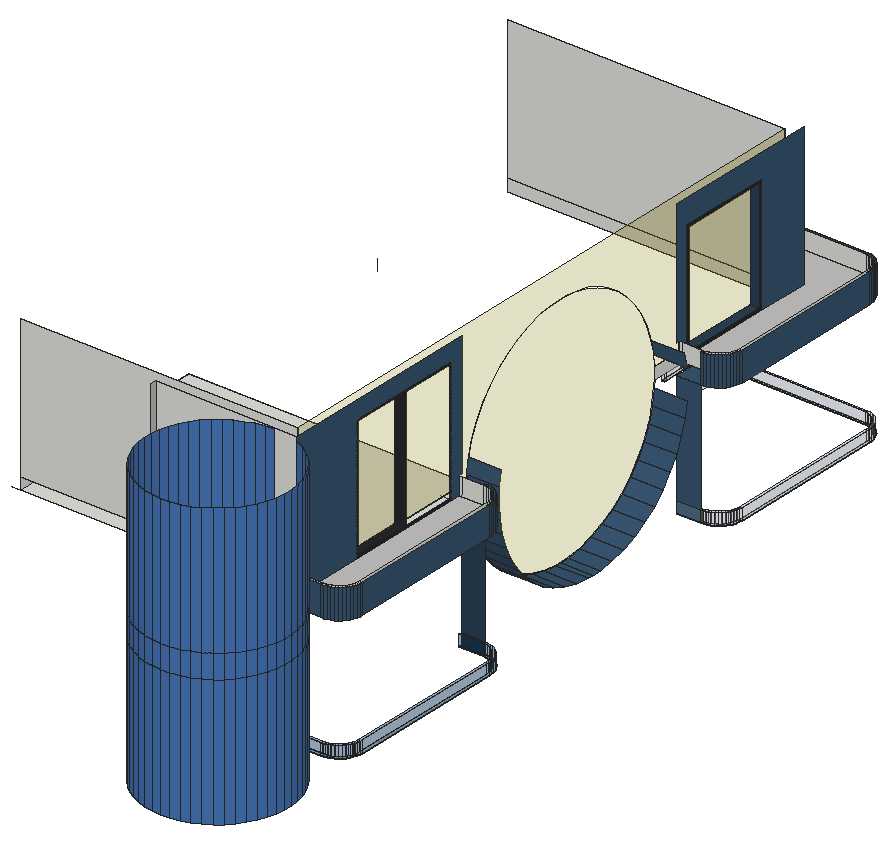
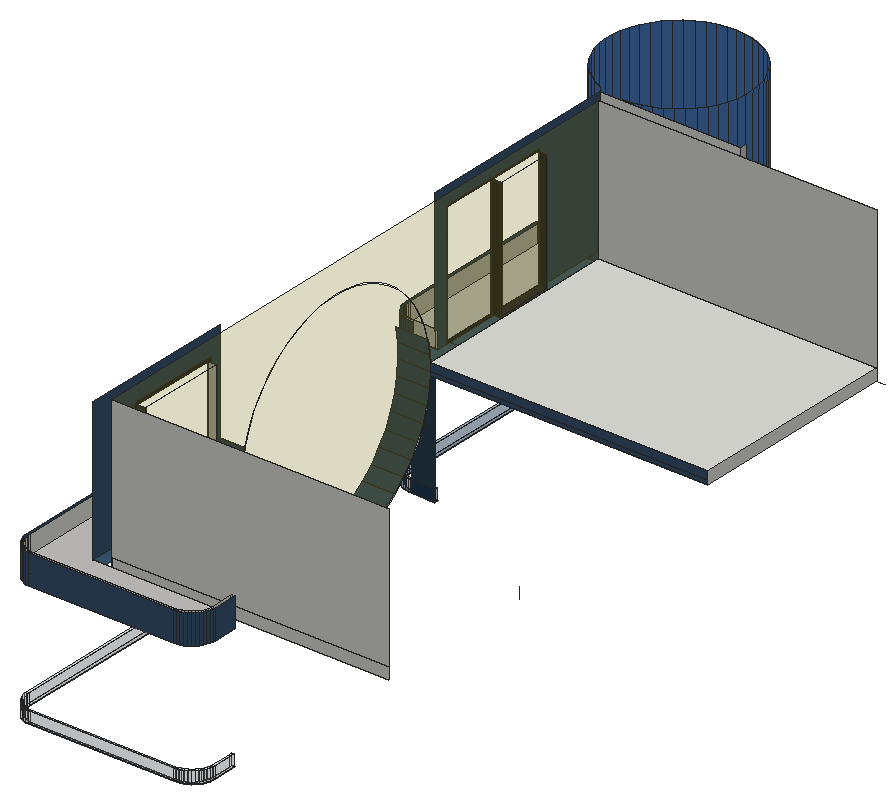
# SketchUp Ruby script. Lengths in inches.
U = 1.inch
M = Sketchup.active_model
def pt(a) = Geom::Point3d.new(a.map { |v| v * U })
def face(e, loops, mat)
  f = e.add_face(loops[0].map { |a| pt(a) })
  loops[1..].each { |l| e.add_face(l.map { |a| pt(a) }).erase! }
  f.material = f.back_material = mat if mat
  f
end
# faces: each face lists its corners as indices into pts; further lists are holes
def faces(e, pts, list, mat = nil) = list.each { |f| face(e, (f[0].is_a?(Array) ? f : [f]).map { |l| l.map { |i| pts[i] } }, mat) }
# xy, xz, yz: faces in a plane at the given z, y or x. An outline is a flat list of corners, or four numbers for a rectangle; further outlines are holes
def ring(l) = l.size == 4 ? [[l[0], l[1]], [l[2], l[1]], [l[2], l[3]], [l[0], l[3]]] : l.each_slice(2).to_a
def flat(e, list, mat, &to3) = list.each { |f| face(e, (f[0].is_a?(Array) ? f : [f]).map { |l| ring(l).map { |u, v| to3.(u, v) } }, mat) }
def xy(e, z, list, mat = nil) = flat(e, list, mat) { |x, y| [x, y, z] }
def xz(e, y, list, mat = nil) = flat(e, list, mat) { |x, z| [x, y, z] }
def yz(e, x, list, mat = nil) = flat(e, list, mat) { |y, z| [x, y, z] }
def lines(e, pts, list) = list.each { |a, b| e.add_line(pt(pts[a]), pt(pts[b])) }
# prism: a flat outline (further loops are holes) pulled along v
def prism(e, loops, v, mat = nil)
  f = face(e, loops, mat); d = Geom::Vector3d.new(v.map { |x| x * U })
  f.pushpull(f.normal.samedirection?(d) ? d.length : -d.length)
end
def box(e, o, s, mat = nil) = prism(e, [[o, [o[0] + s[0], o[1], o[2]], [o[0] + s[0], o[1] + s[1], o[2]], [o[0], o[1] + s[1], o[2]]]], [0, 0, s[2]], mat)
def at(x, y, z, deg = 0) = Geom::Transformation.translation(pt([x, y, z])) * Geom::Transformation.rotation(ORIGIN, Z_AXIS, deg.degrees)
def axes(o, x, y, z) = Geom::Transformation.new([*x, 0, *y, 0, *z, 0, *pt(o).to_a, 1])
def part(name) = M.definitions.add(name)
# library, detail: a bought-in or finely detailed component or shape, given as its bounding box
def library(name, o, s) = part(name).tap { |d| box(d.entities, o, s) }
def detail(e, o, s) = box(e.add_group.entities, o, s)
def put(e, d, t, mat = nil) = e.add_instance(d, t).tap { |i| i.material = mat if mat }
def group(e, t, mat = nil) = e.add_group.tap { |g| g.transformation = t; g.material = mat if mat }.entities
root = M.entities
M.materials.add("Carpet_01_1K").color = [196, 195, 193]
M.materials.add("Carpet_04_1K").color = [56, 85, 112]
M.materials.add("Carpet_04_1K1").color = [43, 65, 85]
M.materials.add("Glass_Basic_01").color = [186, 175, 28]
M.materials["Glass_Basic_01"].alpha = 0.25
M.materials.add("Glass_Basic_1").color = [0, 47, 91]
M.materials["Glass_Basic_1"].alpha = 0.25
M.materials.add("Glass_Basic_2").color = [161, 173, 186]
M.materials["Glass_Basic_2"].alpha = 0.25
M.materials.add("Glass_Mirror_01").color = [71, 118, 185]
M.materials.add("ThomThom - Buttons2").color = [40, 40, 43]
c1 = part("Group\#2")
prism(c1.entities,[[[147,3,0],[168,3,0],[170.74,3.18,0],[173.44,3.72,0],[176.04,4.6,0],[178.5,5.8125,0],[180.78,7.34,0],[182.85,9.15,0],[184.66,11.22,0],[186.1875,13.5,0],[187.4,15.96,0],[188.28,18.56,0],[188.82,21.26,0],[189,24,0],[189,184.94,0],[188.8125,187.78,0],[188.28,190.47,0],[187.4,193.07,0],[186.18,195.54,0],[184.66,197.82,0],[182.84,199.88,0],[180.78,201.7,0],[178.5,203.22,0],[176.03,204.4375,0],[173.43,205.32,0],[171.01,205.8,0],[24,205.8,0],[21.26,205.62,0],[18.56,205.08,0],[15.96,204.2,0],[13.5,202.99,0],[11.22,201.46,0],[9.15,199.65,0],[7.34,197.58,0],[5.8125,195.3,0],[4.6,192.84,0],[3.72,190.24,0],[3.18,187.54,0],[3,184.8,0],[3,163.8,0],[3,160.8,0],[0,160.8,0],[0,184.8,0],[0.21,187.93,0],[0.82,191.01,0],[1.83,193.98,0],[3.22,196.8,0],[4.96,199.41,0],[7.03,201.77,0],[9.39,203.84,0],[12,205.58,0],[14.82,206.97,0],[17.79,207.98,0],[20.87,208.59,0],[24,208.8,0],[171.31,208.8,0],[174.21,208.22,0],[177.18,207.21,0],[180,205.82,0],[182.61,204.08,0],[184.97,202.01,0],[187.04,199.65,0],[188.78,197.04,0],[190.17,194.22,0],[191.18,191.25,0],[191.79,188.17,0],[192,185.04,0],[192,24,0],[191.79,20.87,0],[191.18,17.79,0],[190.17,14.82,0],[188.78,12,0],[187.04,9.39,0],[184.97,7.03,0],[182.61,4.96,0],[180,3.22,0],[177.18,1.83,0],[174.21,0.82,0],[171.13,0.21,0],[168,0,0],[144,0,0],[144,3,0]]],[0,0,12])
c2 = part("Group\#1")
prism(c2.entities,[[[0,206.04,0],[0,209.04,0],[24,209.04,0],[24.001,209.04,0],[27.133,208.835,0],[30.212,208.222,0],[33.184,207.213,0],[36,205.825,0],[38.61,204.081,0],[40.971,202.011,0],[43.04,199.65,0],[44.785,197.04,0],[46.173,194.224,0],[47.182,191.252,0],[47.795,188.173,0],[48,185.04,0],[48,24,0],[47.795,20.867,0],[47.182,17.788,0],[46.602,16.08,0],[46.173,14.816,0],[44.785,12,0],[43.04,9.39,0],[40.971,7.029,0],[38.61,4.96,0],[36,3.215,0],[33.184,1.827,0],[30.212,0.818,0],[27.133,0.205,0],[24,0,0],[0,0,0],[0,3,0],[3,3,0],[24,3,0],[26.741,3.18,0],[29.435,3.716,0],[32.036,4.599,0],[34.5,5.814,0],[36.784,7.34,0],[38.849,9.151,0],[40.66,11.216,0],[42.187,13.5,0],[43.401,15.964,0],[44.284,18.565,0],[44.82,21.259,0],[45,24,0],[45,185.04,0],[44.82,187.781,0],[44.284,190.475,0],[43.401,193.076,0],[42.187,195.54,0],[40.66,197.824,0],[38.849,199.889,0],[36.784,201.701,0],[34.5,203.227,0],[32.036,204.442,0],[29.435,205.325,0],[26.741,205.86,0],[24,206.04,0],[3,206.04,0]]],[0,0,12])
xy(root,636,[[330.57,155.5,354.57,155.5,357.71,155.71,360.79,156.32,363.76,157.33,366.57,158.72,369.19,160.46,371.55,162.53,373.62,164.89,375.36,167.5,376.75,170.32,377.76,173.29,378.37,176.37,378.57,179.5,378.57,340.54,378.37,343.67,377.76,346.75,376.75,349.73,375.36,352.54,373.62,355.15,371.55,357.51,369.19,359.58,366.57,361.33,363.76,362.71,360.79,363.72,357.71,364.34,354.57,364.54,330.57,364.54,330.57,361.54,354.57,361.54,357.32,361.36,360.01,360.83,362.61,359.94,365.07,358.73,367.36,357.2,369.42,355.39,371.24,353.33,372.76,351.04,373.98,348.58,374.86,345.98,375.4,343.28,375.57,340.54,375.57,179.5,375.4,176.76,374.86,174.07,373.98,171.46,372.76,169,371.24,166.72,369.42,164.65,367.36,162.84,365.07,161.31,362.61,160.1,360.01,159.22,357.32,158.68,354.57,158.5,330.57,158.5],[330.57,637.9,354.57,637.9,357.71,638.11,360.79,638.72,363.76,639.73,366.57,641.12,369.19,642.86,371.55,644.93,373.62,647.29,375.36,649.9,376.75,652.72,377.76,655.6875,378.37,658.77,378.57,661.9,378.57,822.94,378.37,826.07,377.76,829.15,376.75,832.125,375.36,834.94,373.62,837.55,371.55,839.91,369.19,841.98,366.57,843.73,363.76,845.11,360.79,846.12,357.88,846.7,210.57,846.7,207.44,846.5,204.36,845.88,201.39,844.875,198.57,843.49,195.96,841.74,193.6,839.67,191.53,837.3125,189.79,834.7,188.4,831.89,187.39,828.91,186.78,825.83,186.57,822.7,186.57,798.7,189.57,798.7,189.57,822.7,189.75,825.44,190.29,828.14,191.17,830.74,192.39,833.2,193.91,835.48,195.73,837.55,197.79,839.36,200.07,840.89,202.54,842.1,205.14,842.99,207.83,843.52,210.57,843.7,357.59,843.7,360.01,843.22,362.61,842.34,365.07,841.12,367.36,839.6,369.42,837.79,371.23,835.72,372.76,833.4375,373.97,830.97,374.85,828.375,375.39,825.68,375.57,822.84,375.57,661.9,375.4,659.16,374.86,656.47,373.98,653.86,372.76,651.4,371.24,649.12,369.42,647.05,367.36,645.24,365.07,643.71,362.61,642.5,360.01,641.62,357.32,641.08,354.57,640.9,330.57,640.9]])
xy(root,735,[[321.57,652.9,330.57,742.9]])
xy(root,742,[[321.57,233.15,330.57,291.15],[321.57,293.15,330.57,349.15]],"ThomThom - Buttons2")
xy(root,762,[[39.57,167.5625,321.57,381.55]])
xy(root,762,[[330.57,155.5,330.57,364.54,354.57,364.54,357.71,364.34,360.79,363.72,363.76,362.71,366.57,361.33,369.19,359.58,371.55,357.51,373.62,355.15,375.36,352.54,376.75,349.73,377.76,346.75,378.37,343.67,378.57,340.54,378.57,179.5,378.37,176.37,377.76,173.29,376.75,170.32,375.36,167.5,373.62,164.89,371.55,162.53,369.19,160.46,366.57,158.72,363.76,157.33,360.79,156.32,357.71,155.71,354.57,155.5],[330.57,637.9,330.57,798.7,186.57,798.7,186.57,822.7,186.78,825.83,187.39,828.91,188.4,831.89,189.79,834.7,191.53,837.3125,193.6,839.67,195.96,841.74,198.57,843.49,201.39,844.875,204.36,845.88,207.44,846.5,210.57,846.7,357.88,846.7,360.79,846.12,363.76,845.11,366.57,843.73,369.19,841.98,371.55,839.91,373.62,837.55,375.36,834.94,376.75,832.125,377.76,829.15,378.37,826.07,378.57,822.94,378.57,661.9,378.37,658.77,377.76,655.6875,376.75,652.72,375.36,649.9,373.62,647.29,371.55,644.93,369.19,642.86,366.57,641.12,363.76,639.73,360.79,638.72,357.71,638.11,354.57,637.9]],"Carpet_04_1K")
xy(root,774,[[39.57,167.5625,321.57,381.61]])
xy(root,774,[[330.57,158.5,354.57,158.5,357.32,158.68,360.01,159.22,362.61,160.1,365.07,161.31,367.36,162.84,369.42,164.65,371.24,166.72,372.76,169,373.98,171.46,374.86,174.07,375.4,176.76,375.57,179.5,375.57,340.54,375.4,343.28,374.86,345.98,373.98,348.58,372.76,351.04,371.24,353.33,369.42,355.39,367.36,357.2,365.07,358.73,362.61,359.94,360.01,360.83,357.32,361.36,354.57,361.54,330.57,361.54],[330.57,640.9,354.57,640.9,357.32,641.08,360.01,641.62,362.61,642.5,365.07,643.71,367.36,645.24,369.42,647.05,371.24,649.12,372.76,651.4,373.98,653.86,374.86,656.47,375.4,659.16,375.57,661.9,375.57,822.84,375.39,825.68,374.85,828.375,373.97,830.97,372.76,833.4375,371.23,835.72,369.42,837.79,367.36,839.6,365.07,841.12,362.61,842.34,360.01,843.22,357.59,843.7,210.57,843.7,207.83,843.52,205.14,842.99,202.54,842.1,200.07,840.89,197.79,839.36,195.73,837.55,193.91,835.48,192.39,833.2,191.17,830.74,190.29,828.14,189.75,825.44,189.57,822.7,189.57,798.7,330.57,798.7]],"Carpet_01_1K")
xy(root,776,[[321.57,233.15,330.57,291.15]],"ThomThom - Buttons2")
xy(root,777,[[321.57,652.9,330.57,742.9]],"Carpet_04_1K1")
xz(root,155.5,[[186.57,762,330.57,774],[186.57,774,330.57,918]])
xz(root,155.5,[[330.57,762,354.57,792]],"Carpet_04_1K")
xz(root,158.5,[[330.57,774,333.57,792],[333.57,774,354.57,792]])
xz(root,167.5625,[[39.57,774,321.57,918]])
xz(root,233.15,[[321.57,776,330.57,898]],"ThomThom - Buttons2")
xz(root,291.15,[[321.57,776,330.57,898]],"ThomThom - Buttons2")
xz(root,293.15,[[321.57,776,330.57,898]],"ThomThom - Buttons2")
xz(root,361.54,[[330.57,774,333.57,792],[333.57,774,354.57,792]])
xz(root,364.54,[[330.57,636,354.57,762]],"Carpet_04_1K1")
xz(root,637.9,[[330.57,636,354.57,762]],"Carpet_04_1K")
xz(root,640.9,[[330.57,774,333.57,791.9],[333.57,774,354.57,791.9]])
xz(root,652.9,[[321.57,777,330.57,891]])
xz(root,742.9,[[321.57,777,330.57,891]],"Carpet_04_1K1")
xz(root,786.64,[[39.57,762,321.57,774],[39.57,774,321.57,918]])
xz(root,843.7,[[210.57,774,357.59,791.9]])
xz(root,846.7,[[210.57,762,357.88,791.9]],"Carpet_04_1K")
yz(root,39.57,[[167.5625,762,381.55,762,381.24,765.87,381.61,774,167.5625,774]])
yz(root,186.57,[[149.51,762,155.5,774],[149.51,774,155.5,918]],"Carpet_01_1K")
yz(root,186.57,[[798.7,762,822.7,791.9]],"Carpet_04_1K")
yz(root,189.57,[[798.7,774,801.7,791.9],[801.7,774,822.7,791.9]])
yz(root,236.92,[[77.22,630,86.26,762],[77.22,762,86.26,786],[77.22,786,86.26,918]],"Glass_Mirror_01")
yz(root,321.57,[[497.02,647.81,482.02,649.28,467.33,652.62,453.17,657.78,439.76,664.67,427.33,673.18,416.0625,683.1875,406.14,694.53,397.71,707.02,390.92,720.47,385.87,734.67,385.57,736,390.45,721.85,397.11,708.33,405.41,695.75,415.22,684.32,426.38,674.2,438.73,665.56,452.0625,658.53,466.17,653.23,480.83,649.75,495.8125,648.12,501.22,648.22,510.88,648.39,525.79,650.54,540.32,654.55,554.23,660.34,567.31,667.84,579.34,676.91,590.14,687.42,599.54,699.2,607.39,712.0625,613.56,725.8125,614.22,727.97,613.98,726.68,607.94,712.87,600.23,699.93,590.95,688.05,580.25,677.43,568.3125,668.24,555.3125,660.62,541.46,654.68,526.98,650.53,512.08,648.23,501.22,647.92],[614.22,727.97,620.93,764.16,620.93,773.73,620.91,774,786.64,774,786.64,762,620.84,762,620.52,755.07,617.96,740.22],[385.28,737.31,382.63,749.39,382.53,750.46],[381.6,774,381.8,779.46,381.875,779.95,381.61,774],[620.89,774,620.74,775.85,620.91,774],
  [619.82,785.95,619.49,787.54,619.8125,786.08]])
yz(root,321.57,[[495.8125,648.12,480.83,649.75,466.17,653.23,452.0625,658.53,438.73,665.56,426.38,674.2,415.22,684.32,405.41,695.75,397.11,708.33,390.45,721.85,385.57,736,385.28,737.31,382.53,750.46,382.09,755.37,381.55,762,381.51,762,381.59,773.73,381.6,774,381.61,774,381.875,779.95,383.82,791.9375,384.27,794.54,388.46,808.79,394.5,822.6,402.22,835.54,411.49,847.41,422.1875,858.03,434.13,867.23,447.13,874.85,460.98,880.78,475.47,884.9375,490.36,887.24,501.22,887.54,505.42,887.66,520.42,886.1875,535.12,882.85,549.28,877.69,562.68,870.8,575.11,862.29,586.38,852.28,596.3,840.9375,604.73,828.44,611.52,814.99,616.58,800.8,619.49,787.54,619.82,785.95,620.74,775.85,620.89,774,620.91,774,620.93,773.73,620.93,764.16,614.22,727.97,613.56,725.8125,607.39,712.0625,599.54,699.2,590.14,687.42,579.34,676.91,567.31,667.84,554.23,660.34,540.32,654.55,525.79,650.54,510.88,648.39,501.22,648.22],[382.09,755.37,381.51,761.73,381.51,762,381.55,762],[[167.5625,774,167.5625,918,786.64,918,786.64,774,620.91,774,620.74,775.85,619.99,785.15,619.82,785.95,619.8125,786.08,619.49,787.54,616.9,799.9,611.99,814.15,605.34,827.67,597.04,840.25,587.23,851.68,576.06,861.8,563.71,870.44,550.38,877.47,536.27,882.77,521.61,886.25,506.63,887.88,501.22,887.78,491.5625,887.61,476.65,885.46,462.12,881.45,448.21,875.66,435.13,868.16,423.1,859.09,412.3,848.58,402.9,836.8,395.06,823.9375,388.88,810.1875,384.48,795.78,384.27,794.54,384.21,794.33,383.82,791.9375,381.92,780.93,381.875,779.95,381.8,779.46,381.6,774],[652.9,777,742.9,891],[233.15,776,291.15,898]],[233.15,776,291.15,898],[652.9,777,742.9,891]],"Glass_Basic_01")
yz(root,330.57,[[158.5,774,231.15,774,231.15,900,351.15,900,351.15,774,361.54,774,361.54,792,364.54,792,364.54,918,155.5,918,155.5,792,158.5,792],[640.9,774,649.9,774,649.9,894,745.9,894,745.9,774,798.7,774,798.7,918,637.9,918,637.9,791.9,640.9,791.9]],"Carpet_04_1K")
yz(root,330.57,[[[231.15,774,351.15,900],[233.15,776,233.15,898,349.15,898,349.15,776,293.15,776,293.15,898,291.15,898,291.15,776]],[[649.9,774,745.9,894],[652.9,777,742.9,891]]],"ThomThom - Buttons2")
yz(root,375.57,[[179.5,774,340.54,792],[661.9,774,822.84,791.9]])
yz(root,378.57,[[179.5,762,340.54,792],[661.9,762,822.94,791.9]],"Carpet_04_1K")
yz(root,380.64,[[77.22,630,86.26,762],[77.22,762,86.26,786],[77.22,786,86.26,918]],"Glass_Mirror_01")
p = [[299.76,10.31,762],[299.76,10.31,630],[308.78,9.74,630],[308.78,9.74,762],[317.8,10.31,630],[317.8,10.31,762],
  [290.875,12,762],[290.875,12,630],[326.6875,12,630],[326.6875,12,762],[282.28,14.79,762],[282.28,14.79,630],
  [335.29,14.79,630],[335.29,14.79,762],[274.09,18.64,762],[274.09,18.64,630],[343.47,18.64,630],[343.47,18.64,762],
  [266.46,23.49,762],[266.46,23.49,630],[351.1,23.49,630],[351.1,23.49,762],[259.49,29.25,762],[259.49,29.25,630],
  [358.07,29.25,630],[358.07,29.25,762],[253.3,35.84,762],[253.3,35.84,630],[364.26,35.84,630],[364.26,35.84,762],
  [247.99,43.16,762],[247.99,43.16,630],[369.57,43.16,630],[369.57,43.16,762],[243.63,51.08,762],[243.63,51.08,630],
  [373.93,51.08,630],[373.93,51.08,762],[240.3,59.49,762],[240.3,59.49,630],[377.26,59.49,630],[377.26,59.49,762],
  [238.06,68.25,762],[238.06,68.25,630],[379.51,68.25,630],[379.51,68.25,762],[236.92,77.22,762],[236.92,77.22,630],
  [380.64,77.22,630],[380.64,77.22,762],[238.06,95.23,762],[238.06,95.23,630],[236.92,86.26,630],[236.92,86.26,762],
  [380.64,86.26,762],[380.64,86.26,630],[379.51,95.23,630],[379.51,95.23,762],[240.3,103.99,762],[240.3,103.99,630],
  [377.26,103.99,630],[377.26,103.99,762],[243.63,112.39,762],[243.63,112.39,630],[373.93,112.39,630],[373.93,112.39,762],
  [247.99,120.32,762],[247.99,120.32,630],[369.57,120.32,630],[369.57,120.32,762],[253.3,127.63,762],[253.3,127.63,630],
  [364.26,127.63,630],[364.26,127.63,762],[259.49,134.22,762],[259.49,134.22,630],[358.07,134.22,630],[358.07,134.22,762],
  [266.46,139.99,762],[266.46,139.99,630],[351.1,139.99,630],[351.1,139.99,762],[274.09,144.83,762],[274.09,144.83,630],
  [343.47,144.83,630],[343.47,144.83,762],[282.28,148.68,762],[282.28,148.68,630],[335.29,148.68,630],[335.29,148.68,762],
  [290.875,151.48,762],[290.875,151.48,630],[299.76,153.17,762],[299.76,153.17,630],[308.78,153.74,762],[308.78,153.74,630],
  [321.57,480.83,649.75],[354.57,480.83,649.75],[354.57,495.8125,648.12],[321.57,495.8125,648.12],[354.57,501.22,648.22],[321.57,501.22,648.22],
  [354.57,510.88,648.39],[321.57,510.88,648.39],[354.57,525.79,650.54],[321.57,525.79,650.54],[321.57,466.17,653.23],[354.57,466.17,653.23],
  [354.57,540.32,654.55],[321.57,540.32,654.55],[321.57,452.0625,658.53],[354.57,452.0625,658.53],[354.57,554.23,660.34],[321.57,554.23,660.34],
  [321.57,438.73,665.56],[354.57,438.73,665.56],[354.57,567.31,667.84],[321.57,567.31,667.84],[321.57,426.38,674.2],[354.57,426.38,674.2],
  [354.57,579.34,676.91],[321.57,579.34,676.91],[321.57,415.22,684.32],[354.57,415.22,684.32],[354.57,590.14,687.42],[321.57,590.14,687.42],
  [321.57,405.41,695.75],[354.57,405.41,695.75],[354.57,599.54,699.2],[321.57,599.54,699.2],[321.57,397.11,708.33],[354.57,397.11,708.33],
  [354.57,607.39,712.0625],[321.57,607.39,712.0625],[321.57,390.45,721.85],[354.57,390.45,721.85],[354.57,613.56,725.8125],[321.57,613.56,725.8125],
  [321.57,385.54,736.1],[354.57,385.54,736.1],[321.57,385.57,736],[354.57,617.96,740.22],[321.57,617.96,740.22],[321.57,614.22,727.97],
  [321.57,382.45,750.85],[354.57,382.45,750.85],[321.57,385.28,737.31],[321.57,382.53,750.46],[354.57,620.52,755.07],[321.57,620.52,755.07],
  [39.57,381.24,765.87],[354.57,381.24,765.87],[321.57,382.09,755.37],[321.57,381.55,762],[39.57,381.55,762],[308.78,9.74,786],
  [299.76,10.31,786],[317.8,10.31,786],[290.875,12,786],[326.6875,12,786],[282.28,14.79,786],[335.29,14.79,786],
  [274.09,18.64,786],[343.47,18.64,786],[266.46,23.49,786],[351.1,23.49,786],[259.49,29.25,786],[358.07,29.25,786],
  [253.3,35.84,786],[364.26,35.84,786],[247.99,43.16,786],[369.57,43.16,786],[243.63,51.08,786],[373.93,51.08,786],
  [240.3,59.49,786],[377.26,59.49,786],[238.06,68.25,786],[379.51,68.25,786],[236.92,77.22,786],[380.64,77.22,786],
  [236.92,86.26,786],[238.06,95.23,786],[379.51,95.23,786],[380.64,86.26,786],[240.3,103.99,786],[377.26,103.99,786],
  [243.63,112.39,786],[373.93,112.39,786],[247.99,120.32,786],[369.57,120.32,786],[253.3,127.63,786],[364.26,127.63,786],
  [259.49,134.22,786],[358.07,134.22,786],[266.46,139.99,786],[351.1,139.99,786],[274.09,144.83,786],[343.47,144.83,786],
  [282.28,148.68,786],[335.29,148.68,786],[290.875,151.48,786],[299.76,153.17,786],[308.78,153.74,786],[357.71,155.71,762],
  [357.71,155.71,792],[354.57,155.5,792],[354.57,155.5,762],[360.79,156.32,762],[360.79,156.32,792],[363.76,157.33,762],
  [363.76,157.33,792],[366.57,158.72,762],[366.57,158.72,792],[369.19,160.46,762],[369.19,160.46,792],[371.55,162.53,762],
  [371.55,162.53,792],[373.62,164.89,762],[373.62,164.89,792],[375.36,167.5,762],[375.36,167.5,792],[376.75,170.32,762],
  [376.75,170.32,792],[377.76,173.29,762],[377.76,173.29,792],[378.37,176.37,762],[378.37,176.37,792],[378.57,179.5,762],
  [378.57,179.5,792],[378.37,343.67,762],[378.37,343.67,792],[378.57,340.54,792],[378.57,340.54,762],[377.76,346.75,762],
  [377.76,346.75,792],[376.75,349.73,762],[376.75,349.73,792],[375.36,352.54,762],[375.36,352.54,792],[373.62,355.15,762],
  [373.62,355.15,792],[371.55,357.51,762],[371.55,357.51,792],[369.19,359.58,762],[369.19,359.58,792],[366.57,361.33,762],
  [366.57,361.33,792],[363.76,362.71,762],[363.76,362.71,792],[360.79,363.72,762],[360.79,363.72,792],[357.71,364.34,762],
  [357.71,364.34,792],[354.57,364.54,762],[354.57,364.54,792],[357.71,638.11,762],[357.71,638.11,791.9],[354.57,637.9,791.9],
  [354.57,637.9,762],[360.79,638.72,762],[360.79,638.72,791.9],[363.76,639.73,762],[363.76,639.73,791.9],[366.57,641.12,762],
  [366.57,641.12,791.9],[369.19,642.86,762],[369.19,642.86,791.9],[371.55,644.93,762],[371.55,644.93,791.9],[373.62,647.29,762],
  [373.62,647.29,791.9],[375.36,649.9,762],[375.36,649.9,791.9],[376.75,652.72,762],[376.75,652.72,791.9],[377.76,655.6875,762],
  [377.76,655.6875,791.9],[378.37,658.77,762],[378.37,658.77,791.9],[378.57,661.9,762],[378.57,661.9,791.9],[186.57,822.7,762],
  [186.57,822.7,791.9],[186.78,825.83,791.9],[186.78,825.83,762],[378.37,826.07,762],[378.37,826.07,791.9],[378.57,822.94,791.9],
  [378.57,822.94,762],[187.39,828.91,791.9],[187.39,828.91,762],[377.76,829.15,762],[377.76,829.15,791.9],[188.4,831.89,791.9],
  [188.4,831.89,762],[376.75,832.125,762],[376.75,832.125,791.9],[189.79,834.7,791.9],[189.79,834.7,762],[375.36,834.94,762],
  [375.36,834.94,791.9],[191.53,837.3125,791.9],[191.53,837.3125,762],[373.62,837.55,762],[373.62,837.55,791.9],[193.6,839.67,791.9],
  [193.6,839.67,762],[371.55,839.91,762],[371.55,839.91,791.9],[195.96,841.74,791.9],[195.96,841.74,762],[369.19,841.98,762],
  [369.19,841.98,791.9],[198.57,843.49,791.9],[198.57,843.49,762],[366.57,843.73,762],[366.57,843.73,791.9],[201.39,844.875,791.9],
  [201.39,844.875,762],[363.76,845.11,762],[363.76,845.11,791.9],[204.36,845.88,791.9],[204.36,845.88,762],[360.79,846.12,762],
  [360.79,846.12,791.9],[207.44,846.5,791.9],[207.44,846.5,762],[357.88,846.7,774],[357.88,846.7,791.9],[357.88,846.7,762],
  [210.57,846.7,791.9],[210.57,846.7,762],[321.57,381.92,780.93],[354.57,381.92,780.93],[39.57,381.61,774],[321.57,381.61,774],
  [321.57,381.875,779.95],[357.32,158.68,774],[354.57,158.5,774],[354.57,158.5,792],[357.32,158.68,792],[360.01,159.22,774],
  [360.01,159.22,792],[362.61,160.1,774],[362.61,160.1,792],[365.07,161.31,774],[365.07,161.31,792],[367.36,162.84,774],
  [367.36,162.84,792],[369.42,164.65,774],[369.42,164.65,792],[371.24,166.72,774],[371.24,166.72,792],[372.76,169,774],
  [372.76,169,792],[373.98,171.46,774],[373.98,171.46,792],[374.86,174.07,774],[374.86,174.07,792],[375.4,176.76,774],
  [375.4,176.76,792],[375.57,179.5,774],[375.57,179.5,792],[375.4,343.28,774],[375.57,340.54,774],[375.57,340.54,792],
  [375.4,343.28,792],[374.86,345.98,774],[374.86,345.98,792],[373.98,348.58,774],[373.98,348.58,792],[372.76,351.04,774],
  [372.76,351.04,792],[371.24,353.33,774],[371.24,353.33,792],[369.42,355.39,774],[369.42,355.39,792],[367.36,357.2,774],
  [367.36,357.2,792],[365.07,358.73,774],[365.07,358.73,792],[362.61,359.94,774],[362.61,359.94,792],[360.01,360.83,774],
  [360.01,360.83,792],[357.32,361.36,774],[357.32,361.36,792],[354.57,361.54,774],[354.57,361.54,792],[357.32,641.08,774],
  [354.57,640.9,774],[354.57,640.9,791.9],[357.32,641.08,791.9],[360.01,641.62,774],[360.01,641.62,791.9],[362.61,642.5,774],
  [362.61,642.5,791.9],[365.07,643.71,774],[365.07,643.71,791.9],[367.36,645.24,774],[367.36,645.24,791.9],[369.42,647.05,774],
  [369.42,647.05,791.9],[371.24,649.12,774],[371.24,649.12,791.9],[372.76,651.4,774],[372.76,651.4,791.9],[373.98,653.86,774],
  [373.98,653.86,791.9],[374.86,656.47,774],[374.86,656.47,791.9],[375.4,659.16,774],[375.4,659.16,791.9],[375.57,661.9,774],
  [375.57,661.9,791.9],[189.57,822.7,774],[189.75,825.44,774],[189.75,825.44,791.9],[189.57,822.7,791.9],[375.39,825.68,774],
  [375.57,822.84,774],[375.57,822.84,791.9],[375.39,825.68,791.9],[190.29,828.14,774],[190.29,828.14,791.9],[374.85,828.375,774],
  [374.85,828.375,791.9],[191.17,830.74,774],[191.17,830.74,791.9],[373.97,830.97,774],[373.97,830.97,791.9],[192.39,833.2,774],
  [192.39,833.2,791.9],[372.76,833.4375,774],[372.76,833.4375,791.9],[193.91,835.48,774],[193.91,835.48,791.9],[371.23,835.72,774],
  [371.23,835.72,791.9],[195.73,837.55,774],[195.73,837.55,791.9],[369.42,837.79,774],[369.42,837.79,791.9],[197.79,839.36,774],
  [197.79,839.36,791.9],[367.36,839.6,774],[367.36,839.6,791.9],[200.07,840.89,774],[200.07,840.89,791.9],[365.07,841.12,774],
  [365.07,841.12,791.9],[202.54,842.1,774],[202.54,842.1,791.9],[362.61,842.34,774],[362.61,842.34,791.9],[205.14,842.99,774],
  [205.14,842.99,791.9],[360.01,843.22,774],[360.01,843.22,791.9],[207.83,843.52,774],[207.83,843.52,791.9],[357.59,843.7,774],
  [357.59,843.7,791.9],[210.57,843.7,774],[210.57,843.7,791.9],[321.57,384.48,795.78],[354.57,384.48,795.78],[321.57,383.82,791.9375],
  [321.57,384.27,794.54],[321.57,619.99,785.15],[354.57,619.99,785.15],[354.57,616.9,799.9],[321.57,616.9,799.9],[321.57,619.49,787.54],
  [321.57,619.82,785.95],[299.76,10.31,918],[308.78,9.74,918],[317.8,10.31,918],[290.875,12,918],[326.6875,12,918],
  [282.28,14.79,918],[335.29,14.79,918],[274.09,18.64,918],[343.47,18.64,918],[266.46,23.49,918],[351.1,23.49,918],
  [259.49,29.25,918],[358.07,29.25,918],[253.3,35.84,918],[364.26,35.84,918],[247.99,43.16,918],[369.57,43.16,918],
  [243.63,51.08,918],[373.93,51.08,918],[240.3,59.49,918],[377.26,59.49,918],[238.06,68.25,918],[379.51,68.25,918],
  [236.92,77.22,918],[380.64,77.22,918],[238.06,95.23,918],[236.92,86.26,918],[380.64,86.26,918],[379.51,95.23,918],
  [240.3,103.99,918],[377.26,103.99,918],[243.63,112.39,918],[373.93,112.39,918],[247.99,120.32,918],[369.57,120.32,918],
  [253.3,127.63,918],[364.26,127.63,918],[259.49,134.22,918],[358.07,134.22,918],[266.46,139.99,918],[351.1,139.99,918],
  [274.09,144.83,918],[343.47,144.83,918],[282.28,148.68,918],[335.29,148.68,918],[290.875,151.48,918],[299.76,153.17,918],
  [308.78,153.74,918],[321.57,786.64,762],[330.57,786.64,762],[39.57,167.5625,762],[30.57,167.5625,762],[321.57,167.5625,762],
  [330.57,167.5625,762],[39.57,620.89,774],[39.57,621.2,770.13],[39.57,620.84,762],[357.71,846.74,774],[354.57,846.94,774],
  [330.57,349.15,776],[321.57,349.15,776],[330.57,150.21,762],[330.57,150.21,786],[330.57,150.21,630]]
faces(root,p,[[0,1,2,3],[3,2,4,5],[6,7,1,0],[5,4,8,9],[10,11,7,6],[9,8,12,13],[14,15,11,10],[13,12,16,17],
  [18,19,15,14],[17,16,20,21],[22,23,19,18],[21,20,24,25],[26,27,23,22],[25,24,28,29],[30,31,27,26],[29,28,32,33],
  [34,35,31,30],[33,32,36,37],[38,39,35,34],[37,36,40,41],[42,43,39,38],[41,40,44,45],[46,47,43,42],[45,44,48,49],
  [50,51,52,53],[54,55,56,57],[58,59,51,50],[57,56,60,61],[62,63,59,58],[61,60,64,65],[66,67,63,62],[65,64,68,69],
  [70,71,67,66],[69,68,72,73],[74,75,71,70],[73,72,76,77],[78,79,75,74],[77,76,80,81],[82,83,79,78],[81,80,84,85],
  [86,87,83,82],[85,84,88,89],[90,91,87,86],[92,93,91,90],[94,95,93,92],[3,155,156,0],[5,157,155,3],[0,156,158,6],
  [9,159,157,5],[6,158,160,10],[13,161,159,9],[10,160,162,14],[17,163,161,13],[14,162,164,18],[21,165,163,17],[18,164,166,22],
  [25,167,165,21],[22,166,168,26],[29,169,167,25],[26,168,170,30],[33,171,169,29],[30,170,172,34],[37,173,171,33],[34,172,174,38],
  [41,175,173,37],[38,174,176,42],[45,177,175,41],[42,176,178,46],[49,179,177,45],[53,180,181,50],[57,182,183,54],[50,181,184,58],
  [61,185,182,57],[58,184,186,62],[65,187,185,61],[62,186,188,66],[69,189,187,65],[66,188,190,70],[73,191,189,69],[70,190,192,74],
  [77,193,191,73],[74,192,194,78],[81,195,193,77],[78,194,196,82],[85,197,195,81],[82,196,198,86],[89,199,197,85],[86,198,200,90],
  [90,200,201,92],[92,201,202,94],[475,156,155,476],[476,155,157,477],[478,158,156,475],[477,157,159,479],[480,160,158,478],[479,159,161,481],
  [482,162,160,480],[481,161,163,483],[484,164,162,482],[483,163,165,485],[486,166,164,484],[485,165,167,487],[488,168,166,486],[487,167,169,489],
  [490,170,168,488],[489,169,171,491],[492,172,170,490],[491,171,173,493],[494,174,172,492],[493,173,175,495],[496,176,174,494],[495,175,177,497],
  [498,178,176,496],[497,177,179,499],[500,181,180,501],[502,183,182,503],[504,184,181,500],[503,182,185,505],[506,186,184,504],[505,185,187,507],
  [508,188,186,506],[507,187,189,509],[510,190,188,508],[509,189,191,511],[512,192,190,510],[511,191,193,513],[514,194,192,512],[513,193,195,515],
  [516,196,194,514],[515,195,197,517],[518,198,196,516],[517,197,199,519],[520,200,198,518],[521,201,200,520],[522,202,201,521]],"Glass_Mirror_01")
faces(root,p,[[96,97,98,99],[99,98,100,101],[101,100,102,103],[103,102,104,105],[106,107,97,96],[105,104,108,109],[110,111,107,106],[109,108,112,113],
  [114,115,111,110],[113,112,116,117],[118,119,115,114],[117,116,120,121],[122,123,119,118],[121,120,124,125],[126,127,123,122],[125,124,128,129],
  [130,131,127,126],[129,128,132,133],[134,135,131,130],[133,132,136,137],[138,139,135,134,140],[137,136,141,142,143],[144,145,139,138,146,147],[142,141,148,149],
  [150,151,145,144,152,153,154],[203,204,205,206],[207,208,204,203],[209,210,208,207],[211,212,210,209],[213,214,212,211],[215,216,214,213],[217,218,216,215],
  [219,220,218,217],[221,222,220,219],[223,224,222,221],[225,226,224,223],[227,228,226,225],[229,230,231,232],[233,234,230,229],[235,236,234,233],
  [237,238,236,235],[239,240,238,237],[241,242,240,239],[243,244,242,241],[245,246,244,243],[247,248,246,245],[249,250,248,247],[251,252,250,249],
  [253,254,252,251],[255,256,257,258],[259,260,256,255],[261,262,260,259],[263,264,262,261],[265,266,264,263],[267,268,266,265],[269,270,268,267],
  [271,272,270,269],[273,274,272,271],[275,276,274,273],[277,278,276,275],[279,280,278,277],[281,282,283,284],[285,286,287,288],[284,283,289,290],
  [291,292,286,285],[290,289,293,294],[295,296,292,291],[294,293,297,298],[299,300,296,295],[298,297,301,302],[303,304,300,299],[302,301,305,306],
  [307,308,304,303],[306,305,309,310],[311,312,308,307],[310,309,313,314],[315,316,312,311],[314,313,317,318],[319,320,316,315],[318,317,321,322],
  [323,324,320,319],[322,321,325,326],[327,328,324,323,329],[326,325,330,331],[332,333,151,150,334,335,336],[465,466,333,332,467,468],[469,470,471,472,473,474]],"Carpet_04_1K")
faces(root,p,[[337,338,339,340],[341,337,340,342],[343,341,342,344],[345,343,344,346],[347,345,346,348],[349,347,348,350],[351,349,350,352],[353,351,352,354],
  [355,353,354,356],[357,355,356,358],[359,357,358,360],[361,359,360,362],[363,364,365,366],[367,363,366,368],[369,367,368,370],[371,369,370,372],
  [373,371,372,374],[375,373,374,376],[377,375,376,378],[379,377,378,380],[381,379,380,382],[383,381,382,384],[385,383,384,386],[387,385,386,388],
  [389,390,391,392],[393,389,392,394],[395,393,394,396],[397,395,396,398],[399,397,398,400],[401,399,400,402],[403,401,402,404],[405,403,404,406],
  [407,405,406,408],[409,407,408,410],[411,409,410,412],[413,411,412,414],[415,416,417,418],[419,420,421,422],[416,423,424,417],[425,419,422,426],
  [423,427,428,424],[429,425,426,430],[427,431,432,428],[433,429,430,434],[431,435,436,432],[437,433,434,438],[435,439,440,436],[441,437,438,442],
  [439,443,444,440],[445,441,442,446],[443,447,448,444],[449,445,446,450],[447,451,452,448],[453,449,450,454],[451,455,456,452],[457,453,454,458],
  [455,459,460,456],[461,457,458,462],[459,463,464,460]])
lines(root,p,[[523,524],[525,526],[527,528],[529,530],[530,531],[532,533],[327,532],[534,535],[89,536],[199,537],[88,538]])
put(root,c1,at(186.57,637.9,636),"Glass_Basic_2")
put(root,c2,at(330.57,155.5,636),"Glass_Basic_1")
